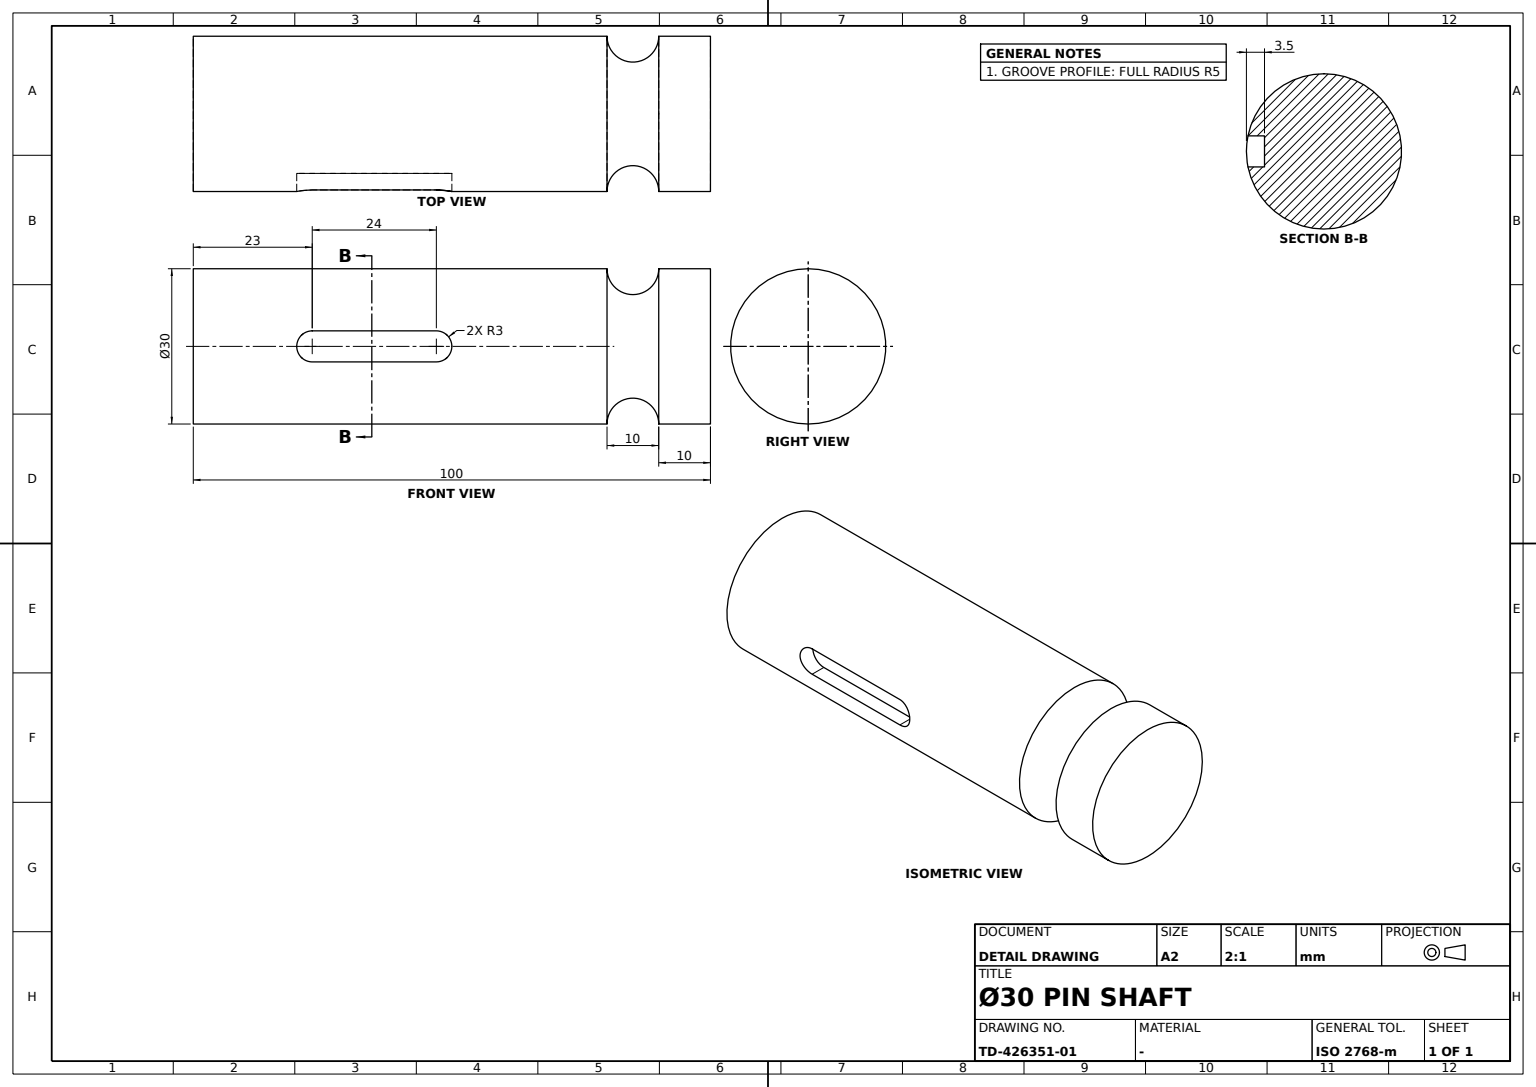
ISO-10303-21;
HEADER;
FILE_DESCRIPTION((''),'2;1');
FILE_NAME('','',(''),(''),'','','');
FILE_SCHEMA(('AUTOMOTIVE_DESIGN'));
ENDSEC;
DATA;
#1=APPLICATION_CONTEXT('');
#2=PRODUCT_CONTEXT('',#1,'mechanical');
#3=PRODUCT('','','',(#2));
#4=PRODUCT_DEFINITION_FORMATION('','',#3);
#5=PRODUCT_DEFINITION_CONTEXT('',#1,'design');
#6=PRODUCT_DEFINITION('','',#4,#5);
#7=PRODUCT_DEFINITION_SHAPE('','',#6);
#8=(LENGTH_UNIT()NAMED_UNIT(*)SI_UNIT(.MILLI.,.METRE.));
#9=(NAMED_UNIT(*)PLANE_ANGLE_UNIT()SI_UNIT($,.RADIAN.));
#10=(NAMED_UNIT(*)SI_UNIT($,.STERADIAN.)SOLID_ANGLE_UNIT());
#11=UNCERTAINTY_MEASURE_WITH_UNIT(LENGTH_MEASURE(0.005),#8,'distance_accuracy_value','');
#12=(GEOMETRIC_REPRESENTATION_CONTEXT(3)GLOBAL_UNCERTAINTY_ASSIGNED_CONTEXT((#11))GLOBAL_UNIT_ASSIGNED_CONTEXT((#8,#9,#10))REPRESENTATION_CONTEXT('',''));
#13=CARTESIAN_POINT('',(14.696938,23.,-3.));
#14=VERTEX_POINT('',#13);
#15=CARTESIAN_POINT('',(11.5,23.,-3.));
#16=VERTEX_POINT('',#15);
#17=CARTESIAN_POINT('',(13.25,23.,-3.));
#18=DIRECTION('',(1.,0.,0.));
#19=VECTOR('',#18,1000.);
#20=LINE('',#17,#19);
#21=EDGE_CURVE('',#14,#16,#20,.F.);
#22=ORIENTED_EDGE('',*,*,#21,.F.);
#23=CARTESIAN_POINT('',(14.696938,47.,-3.));
#24=VERTEX_POINT('',#23);
#25=DIRECTION('',(0.,1.,0.));
#26=VECTOR('',#25,1000.);
#27=LINE('',#13,#26);
#28=EDGE_CURVE('',#14,#24,#27,.T.);
#29=ORIENTED_EDGE('',*,*,#28,.T.);
#30=CARTESIAN_POINT('',(11.5,47.,-3.));
#31=VERTEX_POINT('',#30);
#32=CARTESIAN_POINT('',(13.25,47.,-3.));
#33=LINE('',#32,#19);
#34=EDGE_CURVE('',#24,#31,#33,.F.);
#35=ORIENTED_EDGE('',*,*,#34,.T.);
#36=LINE('',#15,#26);
#37=EDGE_CURVE('',#16,#31,#36,.T.);
#38=ORIENTED_EDGE('',*,*,#37,.F.);
#39=EDGE_LOOP('',(#22,#29,#35,#38));
#40=FACE_BOUND('',#39,.T.);
#41=CARTESIAN_POINT('',(15.,23.,-3.));
#42=DIRECTION('',(0.,0.,1.));
#43=AXIS2_PLACEMENT_3D('',#41,#42,#25);
#44=PLANE('',#43);
#45=ADVANCED_FACE('',(#40),#44,.T.);
#46=CARTESIAN_POINT('',(11.5,23.,3.));
#47=VERTEX_POINT('',#46);
#48=CARTESIAN_POINT('',(11.5,23.,0.));
#49=DIRECTION('',(0.,0.,-1.));
#50=AXIS2_PLACEMENT_3D('',#48,#18,#49);
#51=CIRCLE('',#50,3.);
#52=EDGE_CURVE('',#47,#16,#51,.T.);
#53=ORIENTED_EDGE('',*,*,#52,.T.);
#54=ORIENTED_EDGE('',*,*,#37,.T.);
#55=CARTESIAN_POINT('',(11.5,47.,3.));
#56=VERTEX_POINT('',#55);
#57=CARTESIAN_POINT('',(11.5,47.,0.));
#58=AXIS2_PLACEMENT_3D('',#57,#18,#49);
#59=CIRCLE('',#58,3.);
#60=EDGE_CURVE('',#31,#56,#59,.T.);
#61=ORIENTED_EDGE('',*,*,#60,.T.);
#62=LINE('',#46,#26);
#63=EDGE_CURVE('',#47,#56,#62,.T.);
#64=ORIENTED_EDGE('',*,*,#63,.F.);
#65=EDGE_LOOP('',(#53,#54,#61,#64));
#66=FACE_BOUND('',#65,.T.);
#67=CARTESIAN_POINT('',(11.5,0.,0.));
#68=AXIS2_PLACEMENT_3D('',#67,#18,#25);
#69=PLANE('',#68);
#70=ADVANCED_FACE('',(#66),#69,.T.);
#71=CARTESIAN_POINT('',(0.,0.,15.));
#72=VERTEX_POINT('',#71);
#73=CARTESIAN_POINT('',(0.,0.,0.));
#74=AXIS2_PLACEMENT_3D('',#73,#25,#42);
#75=CIRCLE('',#74,15.);
#76=EDGE_CURVE('',#72,#72,#75,.T.);
#77=ORIENTED_EDGE('',*,*,#76,.T.);
#78=EDGE_LOOP('',(#77));
#79=FACE_BOUND('',#78,.T.);
#80=CARTESIAN_POINT('',(0.,80.,15.));
#81=VERTEX_POINT('',#80);
#82=CARTESIAN_POINT('',(0.,80.,0.));
#83=AXIS2_PLACEMENT_3D('',#82,#25,#42);
#84=CIRCLE('',#83,15.);
#85=EDGE_CURVE('',#81,#81,#84,.T.);
#86=ORIENTED_EDGE('',*,*,#85,.F.);
#87=EDGE_LOOP('',(#86));
#88=FACE_BOUND('',#87,.T.);
#89=CARTESIAN_POINT('',(14.696938,23.,3.));
#90=VERTEX_POINT('',#89);
#91=CARTESIAN_POINT('',(14.696938,22.2055,3.));
#92=CARTESIAN_POINT('',(14.849856,20.655728,2.352145));
#93=CARTESIAN_POINT('',(15.074997,19.672665,-0.000703));
#94=CARTESIAN_POINT('',(14.850155,20.653613,-2.349645));
#95=CARTESIAN_POINT('',(14.696938,22.205536,-3.));
#96=B_SPLINE_CURVE_WITH_KNOTS('',3,(#89,#91,#92,#93,#94,#95,#13),.UNSPECIFIED.,.F.,.F.,(4,1,1,1,4),(-0.004698252,-0.002349101,0.000000051,0.002349203,0.004698354),.UNSPECIFIED.);
#97=EDGE_CURVE('',#90,#14,#96,.T.);
#98=ORIENTED_EDGE('',*,*,#97,.F.);
#99=CARTESIAN_POINT('',(14.696938,47.,3.));
#100=VERTEX_POINT('',#99);
#101=LINE('',#89,#26);
#102=EDGE_CURVE('',#90,#100,#101,.T.);
#103=ORIENTED_EDGE('',*,*,#102,.T.);
#104=CARTESIAN_POINT('',(14.696938,47.7945,-3.));
#105=CARTESIAN_POINT('',(14.849856,49.344272,-2.352145));
#106=CARTESIAN_POINT('',(15.074997,50.327335,0.000703));
#107=CARTESIAN_POINT('',(14.850155,49.346387,2.349645));
#108=CARTESIAN_POINT('',(14.696938,47.794464,3.));
#109=B_SPLINE_CURVE_WITH_KNOTS('',3,(#23,#104,#105,#106,#107,#108,#99),.UNSPECIFIED.,.F.,.F.,(4,1,1,1,4),(-0.004698252,-0.002349101,0.000000051,0.002349203,0.004698354),.UNSPECIFIED.);
#110=EDGE_CURVE('',#24,#100,#109,.T.);
#111=ORIENTED_EDGE('',*,*,#110,.F.);
#112=ORIENTED_EDGE('',*,*,#28,.F.);
#113=EDGE_LOOP('',(#98,#103,#111,#112));
#114=FACE_BOUND('',#113,.T.);
#115=CARTESIAN_POINT('',(0.,50.,0.));
#116=DIRECTION('',(-1.,0.,0.));
#117=AXIS2_PLACEMENT_3D('',#115,#25,#116);
#118=CYLINDRICAL_SURFACE('',#117,15.);
#119=ADVANCED_FACE('',(#79,#88,#114),#118,.T.);
#120=CARTESIAN_POINT('',(0.,90.,15.));
#121=VERTEX_POINT('',#120);
#122=CARTESIAN_POINT('',(0.,90.,0.));
#123=AXIS2_PLACEMENT_3D('',#122,#25,#42);
#124=CIRCLE('',#123,15.);
#125=EDGE_CURVE('',#121,#121,#124,.F.);
#126=ORIENTED_EDGE('',*,*,#125,.T.);
#127=EDGE_LOOP('',(#126));
#128=FACE_BOUND('',#127,.T.);
#129=ORIENTED_EDGE('',*,*,#85,.T.);
#130=EDGE_LOOP('',(#129));
#131=FACE_BOUND('',#130,.T.);
#132=CARTESIAN_POINT('',(0.,85.,0.));
#133=AXIS2_PLACEMENT_3D('',#132,#25,#18);
#134=TOROIDAL_SURFACE('',#133,15.,5.);
#135=ADVANCED_FACE('',(#128,#131),#134,.F.);
#136=ORIENTED_EDGE('',*,*,#110,.T.);
#137=CARTESIAN_POINT('',(13.25,47.,3.));
#138=LINE('',#137,#19);
#139=EDGE_CURVE('',#100,#56,#138,.F.);
#140=ORIENTED_EDGE('',*,*,#139,.T.);
#141=ORIENTED_EDGE('',*,*,#60,.F.);
#142=ORIENTED_EDGE('',*,*,#34,.F.);
#143=EDGE_LOOP('',(#136,#140,#141,#142));
#144=FACE_BOUND('',#143,.T.);
#145=CARTESIAN_POINT('',(13.25,47.,0.));
#146=AXIS2_PLACEMENT_3D('',#145,#18,#25);
#147=CYLINDRICAL_SURFACE('',#146,3.);
#148=ADVANCED_FACE('',(#144),#147,.F.);
#149=ORIENTED_EDGE('',*,*,#21,.T.);
#150=ORIENTED_EDGE('',*,*,#52,.F.);
#151=CARTESIAN_POINT('',(13.25,23.,3.));
#152=LINE('',#151,#19);
#153=EDGE_CURVE('',#90,#47,#152,.F.);
#154=ORIENTED_EDGE('',*,*,#153,.F.);
#155=ORIENTED_EDGE('',*,*,#97,.T.);
#156=EDGE_LOOP('',(#149,#150,#154,#155));
#157=FACE_BOUND('',#156,.T.);
#158=CARTESIAN_POINT('',(13.25,23.,0.));
#159=AXIS2_PLACEMENT_3D('',#158,#18,#25);
#160=CYLINDRICAL_SURFACE('',#159,3.);
#161=ADVANCED_FACE('',(#157),#160,.F.);
#162=ORIENTED_EDGE('',*,*,#76,.F.);
#163=EDGE_LOOP('',(#162));
#164=FACE_BOUND('',#163,.T.);
#165=AXIS2_PLACEMENT_3D('',#73,#25,#116);
#166=PLANE('',#165);
#167=ADVANCED_FACE('',(#164),#166,.F.);
#168=ORIENTED_EDGE('',*,*,#153,.T.);
#169=ORIENTED_EDGE('',*,*,#63,.T.);
#170=ORIENTED_EDGE('',*,*,#139,.F.);
#171=ORIENTED_EDGE('',*,*,#102,.F.);
#172=EDGE_LOOP('',(#168,#169,#170,#171));
#173=FACE_BOUND('',#172,.T.);
#174=CARTESIAN_POINT('',(15.,23.,3.));
#175=AXIS2_PLACEMENT_3D('',#174,#42,#25);
#176=PLANE('',#175);
#177=ADVANCED_FACE('',(#173),#176,.F.);
#178=ORIENTED_EDGE('',*,*,#125,.F.);
#179=EDGE_LOOP('',(#178));
#180=FACE_BOUND('',#179,.T.);
#181=CARTESIAN_POINT('',(0.,100.,15.));
#182=VERTEX_POINT('',#181);
#183=CARTESIAN_POINT('',(0.,100.,0.));
#184=AXIS2_PLACEMENT_3D('',#183,#25,#42);
#185=CIRCLE('',#184,15.);
#186=EDGE_CURVE('',#182,#182,#185,.T.);
#187=ORIENTED_EDGE('',*,*,#186,.F.);
#188=EDGE_LOOP('',(#187));
#189=FACE_BOUND('',#188,.T.);
#190=ADVANCED_FACE('',(#180,#189),#118,.T.);
#191=ORIENTED_EDGE('',*,*,#186,.T.);
#192=EDGE_LOOP('',(#191));
#193=FACE_BOUND('',#192,.T.);
#194=AXIS2_PLACEMENT_3D('',#183,#25,#116);
#195=PLANE('',#194);
#196=ADVANCED_FACE('',(#193),#195,.T.);
#197=CLOSED_SHELL('',(#45,#70,#119,#135,#148,#161,#167,#177,#190,#196));
#198=MANIFOLD_SOLID_BREP('',#197);
#199=ADVANCED_BREP_SHAPE_REPRESENTATION('',(#198),#12);
#200=SHAPE_DEFINITION_REPRESENTATION(#7,#199);
ENDSEC;
END-ISO-10303-21;
